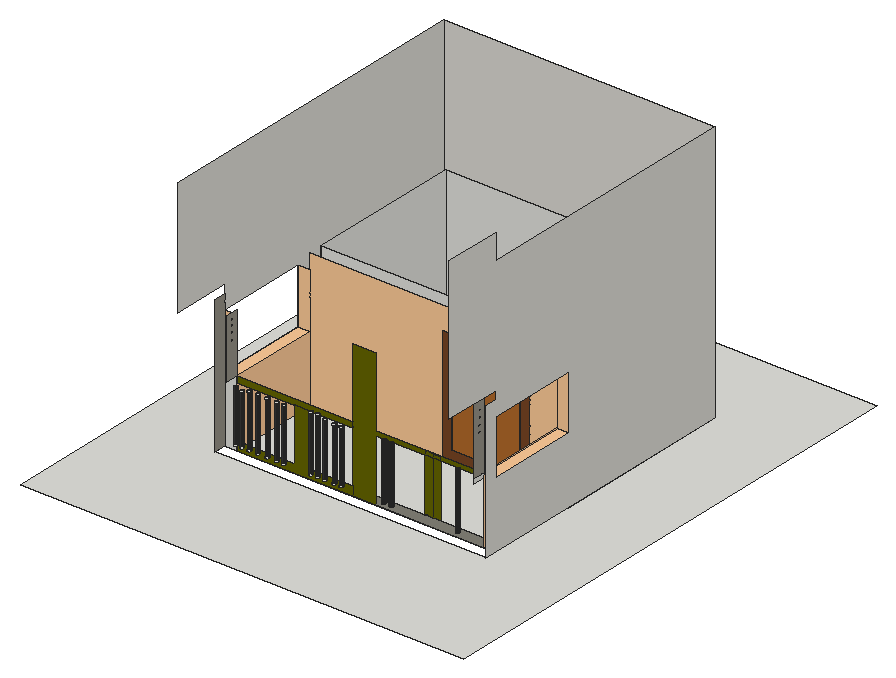
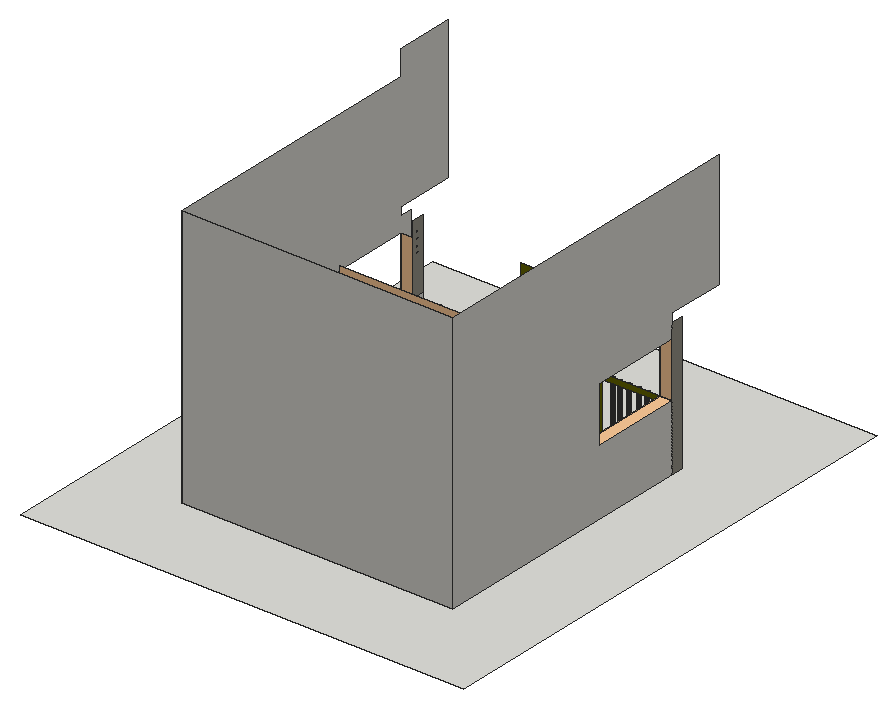
# SketchUp Ruby script. Lengths in inches.
U = 1.inch
M = Sketchup.active_model
def pt(a) = Geom::Point3d.new(a.map { |v| v * U })
def face(e, loops, mat)
  f = e.add_face(loops[0].map { |a| pt(a) })
  loops[1..].each { |l| e.add_face(l.map { |a| pt(a) }).erase! }
  f.material = f.back_material = mat if mat
  f
end
# faces: each face lists its corners as indices into pts; further lists are holes
def faces(e, pts, list, mat = nil) = list.each { |f| face(e, (f[0].is_a?(Array) ? f : [f]).map { |l| l.map { |i| pts[i] } }, mat) }
# xy, xz, yz: faces in a plane at the given z, y or x. An outline is a flat list of corners, or four numbers for a rectangle; further outlines are holes
def ring(l) = l.size == 4 ? [[l[0], l[1]], [l[2], l[1]], [l[2], l[3]], [l[0], l[3]]] : l.each_slice(2).to_a
def flat(e, list, mat, &to3) = list.each { |f| face(e, (f[0].is_a?(Array) ? f : [f]).map { |l| ring(l).map { |u, v| to3.(u, v) } }, mat) }
def xy(e, z, list, mat = nil) = flat(e, list, mat) { |x, y| [x, y, z] }
def xz(e, y, list, mat = nil) = flat(e, list, mat) { |x, z| [x, y, z] }
def yz(e, x, list, mat = nil) = flat(e, list, mat) { |y, z| [x, y, z] }
def lines(e, pts, list) = list.each { |a, b| e.add_line(pt(pts[a]), pt(pts[b])) }
# prism: a flat outline (further loops are holes) pulled along v
def prism(e, loops, v, mat = nil)
  f = face(e, loops, mat); d = Geom::Vector3d.new(v.map { |x| x * U })
  f.pushpull(f.normal.samedirection?(d) ? d.length : -d.length)
end
def box(e, o, s, mat = nil) = prism(e, [[o, [o[0] + s[0], o[1], o[2]], [o[0] + s[0], o[1] + s[1], o[2]], [o[0], o[1] + s[1], o[2]]]], [0, 0, s[2]], mat)
def at(x, y, z, deg = 0) = Geom::Transformation.translation(pt([x, y, z])) * Geom::Transformation.rotation(ORIGIN, Z_AXIS, deg.degrees)
def axes(o, x, y, z) = Geom::Transformation.new([*x, 0, *y, 0, *z, 0, *pt(o).to_a, 1])
def part(name) = M.definitions.add(name)
# library, detail: a bought-in or finely detailed component or shape, given as its bounding box
def library(name, o, s) = part(name).tap { |d| box(d.entities, o, s) }
def detail(e, o, s) = box(e.add_group.entities, o, s)
def put(e, d, t, mat = nil) = e.add_instance(d, t).tap { |i| i.material = mat if mat }
def group(e, t, mat = nil) = e.add_group.tap { |g| g.transformation = t; g.material = mat if mat }.entities
root = M.entities
M.materials.add("[Color C02]").color = [255, 204, 153]
M.materials.add("[Color E08]").color = [102, 102, 0]
M.materials.add("[Color M07]").color = [58, 58, 58]
M.materials.add("[Formica Graystone]").color = [149, 146, 135]
M.materials.add("[Terrazzo Tile Light]").color = [219, 217, 210]
M.materials.add("[Wood Bamboo]").color = [177, 105, 43]
M.materials.add("[Wood Veneer 01]").color = [120, 70, 37]
xy(root,0,[[[0,0,171.0625,199],[33.03,52.46,137.78,162.77]],[33.03,57.16,37.72,92.52],[37.72,57.16,133.09,92.52],[133.09,57.16,137.78,92.52],[[33.03,92.52,137.78,162.77],[37.72,98,133.09,158.08]],
  [37.72,98,133.09,158.08]])
xy(root,3.4375,[[39.18,54.27,39,54.29,38.83,54.36,38.69,54.47,38.58,54.61,38.51,54.78,38.49,54.96,38.51,55.13,38.58,55.3,38.69,55.44,38.83,55.55,39,55.62,39.18,55.64,39.35,55.62,39.52,55.55,39.66,55.44,39.77,55.3,39.84,55.13,39.86,54.96,39.84,54.78,39.77,54.61,39.66,54.47,39.52,54.36,39.35,54.29],[41.55,54.27,41.375,54.29,41.21,54.36,41.07,54.47,40.96,54.61,40.89,54.78,40.86,54.96,40.89,55.13,40.96,55.3,41.07,55.44,41.21,55.55,41.375,55.62,41.55,55.64,41.73,55.62,41.9,55.55,42.04,55.44,42.15,55.3,42.22,55.13,42.24,54.96,42.22,54.78,42.15,54.61,42.04,54.47,41.9,54.36,41.73,54.29],[44.43,54.27,44.25,54.29,44.08,54.36,43.94,54.47,43.83,54.61,43.76,54.78,43.74,54.96,43.76,55.13,43.83,55.3,43.94,55.44,44.08,55.55,44.25,55.62,44.43,55.64,44.6,55.62,44.77,55.55,44.91,55.44,45.02,55.3,45.09,55.13,45.11,54.96,45.09,54.78,45.02,54.61,44.91,54.47,44.77,54.36,44.6,54.29],[47.68,54.27,47.5,54.29,47.33,54.36,47.19,54.47,47.08,54.61,47.01,54.78,46.99,54.96,47.01,55.13,47.08,55.3,47.19,55.44,47.33,55.55,47.5,55.62,47.68,55.64,47.85,55.62,48.02,55.55,48.16,55.44,48.27,55.3,48.34,55.13,48.36,54.96,48.34,54.78,48.27,54.61,48.16,54.47,48.02,54.36,47.85,54.29],[51.36,54.27,51.1875,54.29,51.02,54.36,50.88,54.47,50.77,54.61,50.7,54.78,50.68,54.96,50.7,55.13,50.77,55.3,50.88,55.44,51.02,55.55,51.1875,55.62,51.36,55.64,51.54,55.62,51.71,55.55,51.85,55.44,51.96,55.3,52.03,55.13,52.05,54.96,52.03,54.78,51.96,54.61,51.85,54.47,51.71,54.36,51.54,54.29],
  [54.99,54.27,54.8125,54.29,54.65,54.36,54.5,54.47,54.39,54.61,54.32,54.78,54.3,54.96,54.32,55.13,54.39,55.3,54.5,55.44,54.65,55.55,54.8125,55.62,54.99,55.64,55.17,55.62,55.33,55.55,55.48,55.44,55.58,55.3,55.65,55.13,55.68,54.96,55.65,54.78,55.58,54.61,55.48,54.47,55.33,54.36,55.17,54.29],[57.74,54.27,57.5625,54.29,57.4,54.36,57.25,54.47,57.14,54.61,57.07,54.78,57.05,54.96,57.07,55.13,57.14,55.3,57.25,55.44,57.4,55.55,57.5625,55.62,57.74,55.64,57.92,55.62,58.08,55.55,58.23,55.44,58.33,55.3,58.4,55.13,58.43,54.96,58.4,54.78,58.33,54.61,58.23,54.47,58.08,54.36,57.92,54.29],[68.11,54.27,67.9375,54.29,67.77,54.36,67.63,54.47,67.52,54.61,67.45,54.78,67.43,54.96,67.45,55.13,67.52,55.3,67.63,55.44,67.77,55.55,67.9375,55.62,68.11,55.64,68.29,55.62,68.46,55.55,68.6,55.44,68.71,55.3,68.78,55.13,68.8,54.96,68.78,54.78,68.71,54.61,68.6,54.47,68.46,54.36,68.29,54.29],[70.74,54.27,70.5625,54.29,70.4,54.36,70.25,54.47,70.14,54.61,70.07,54.78,70.05,54.96,70.07,55.13,70.14,55.3,70.25,55.44,70.4,55.55,70.5625,55.62,70.74,55.64,70.92,55.62,71.08,55.55,71.23,55.44,71.33,55.3,71.4,55.13,71.43,54.96,71.4,54.78,71.33,54.61,71.23,54.47,71.08,54.36,70.92,54.29],[73.55,54.27,73.375,54.29,73.21,54.36,73.07,54.47,72.96,54.61,72.89,54.78,72.86,54.96,72.89,55.13,72.96,55.3,73.07,55.44,73.21,55.55,73.375,55.62,73.55,55.64,73.73,55.62,73.9,55.55,74.04,55.44,74.15,55.3,74.22,55.13,74.24,54.96,74.22,54.78,74.15,54.61,74.04,54.47,73.9,54.36,73.73,54.29],
  [77.18,54.27,77,54.29,76.83,54.36,76.69,54.47,76.58,54.61,76.51,54.78,76.49,54.96,76.51,55.13,76.58,55.3,76.69,55.44,76.83,55.55,77,55.62,77.18,55.64,77.35,55.62,77.52,55.55,77.66,55.44,77.77,55.3,77.84,55.13,77.86,54.96,77.84,54.78,77.77,54.61,77.66,54.47,77.52,54.36,77.35,54.29],[79.8,54.27,79.625,54.29,79.46,54.36,79.32,54.47,79.21,54.61,79.14,54.78,79.11,54.96,79.14,55.13,79.21,55.3,79.32,55.44,79.46,55.55,79.625,55.62,79.8,55.64,79.98,55.62,80.15,55.55,80.29,55.44,80.4,55.3,80.47,55.13,80.49,54.96,80.47,54.78,80.4,54.61,80.29,54.47,80.15,54.36,79.98,54.29]])
xy(root,3.82,[[92.4,92.52,118.56,98]])
xy(root,22.875,[[41.55,54.27,41.73,54.29,41.9,54.36,42.04,54.47,42.15,54.61,42.22,54.78,42.24,54.96,42.22,55.13,42.15,55.3,42.04,55.44,41.9,55.55,41.73,55.62,41.55,55.64,41.375,55.62,41.21,55.55,41.07,55.44,40.96,55.3,40.89,55.13,40.86,54.96,40.89,54.78,40.96,54.61,41.07,54.47,41.21,54.36,41.375,54.29]])
xy(root,23.8125,[[54.99,54.27,55.17,54.29,55.33,54.36,55.48,54.47,55.58,54.61,55.65,54.78,55.68,54.96,55.65,55.13,55.58,55.3,55.48,55.44,55.33,55.55,55.17,55.62,54.99,55.64,54.8125,55.62,54.65,55.55,54.5,55.44,54.39,55.3,54.32,55.13,54.3,54.96,54.32,54.78,54.39,54.61,54.5,54.47,54.65,54.36,54.8125,54.29]])
xy(root,23.875,[[44.43,54.27,44.6,54.29,44.77,54.36,44.91,54.47,45.02,54.61,45.09,54.78,45.11,54.96,45.09,55.13,45.02,55.3,44.91,55.44,44.77,55.55,44.6,55.62,44.43,55.64,44.25,55.62,44.08,55.55,43.94,55.44,43.83,55.3,43.76,55.13,43.74,54.96,43.76,54.78,43.83,54.61,43.94,54.47,44.08,54.36,44.25,54.29]])
xy(root,23.9375,[[47.68,54.27,47.85,54.29,48.02,54.36,48.16,54.47,48.27,54.61,48.34,54.78,48.36,54.96,48.34,55.13,48.27,55.3,48.16,55.44,48.02,55.55,47.85,55.62,47.68,55.64,47.5,55.62,47.33,55.55,47.19,55.44,47.08,55.3,47.01,55.13,46.99,54.96,47.01,54.78,47.08,54.61,47.19,54.47,47.33,54.36,47.5,54.29],[51.36,54.27,51.54,54.29,51.71,54.36,51.85,54.47,51.96,54.61,52.03,54.78,52.05,54.96,52.03,55.13,51.96,55.3,51.85,55.44,51.71,55.55,51.54,55.62,51.36,55.64,51.1875,55.62,51.02,55.55,50.88,55.44,50.77,55.3,50.7,55.13,50.68,54.96,50.7,54.78,50.77,54.61,50.88,54.47,51.02,54.36,51.1875,54.29],[57.74,54.27,57.92,54.29,58.08,54.36,58.23,54.47,58.33,54.61,58.4,54.78,58.43,54.96,58.4,55.13,58.33,55.3,58.23,55.44,58.08,55.55,57.92,55.62,57.74,55.64,57.5625,55.62,57.4,55.55,57.25,55.44,57.14,55.3,57.07,55.13,57.05,54.96,57.07,54.78,57.14,54.61,57.25,54.47,57.4,54.36,57.5625,54.29]])
xy(root,24,[[77.18,54.27,77.35,54.29,77.52,54.36,77.66,54.47,77.77,54.61,77.84,54.78,77.86,54.96,77.84,55.13,77.77,55.3,77.66,55.44,77.52,55.55,77.35,55.62,77.18,55.64,77,55.62,76.83,55.55,76.69,55.44,76.58,55.3,76.51,55.13,76.49,54.96,76.51,54.78,76.58,54.61,76.69,54.47,76.83,54.36,77,54.29]])
xy(root,24.0625,[[79.8,54.27,79.98,54.29,80.15,54.36,80.29,54.47,80.4,54.61,80.47,54.78,80.49,54.96,80.47,55.13,80.4,55.3,80.29,55.44,80.15,55.55,79.98,55.62,79.8,55.64,79.625,55.62,79.46,55.55,79.32,55.44,79.21,55.3,79.14,55.13,79.11,54.96,79.14,54.78,79.21,54.61,79.32,54.47,79.46,54.36,79.625,54.29]])
xy(root,24.375,[[73.55,54.27,73.73,54.29,73.9,54.36,74.04,54.47,74.15,54.61,74.22,54.78,74.24,54.96,74.22,55.13,74.15,55.3,74.04,55.44,73.9,55.55,73.73,55.62,73.55,55.64,73.375,55.62,73.21,55.55,73.07,55.44,72.96,55.3,72.89,55.13,72.86,54.96,72.89,54.78,72.96,54.61,73.07,54.47,73.21,54.36,73.375,54.29]])
xy(root,25.0625,[[68.11,54.27,68.29,54.29,68.46,54.36,68.6,54.47,68.71,54.61,68.78,54.78,68.8,54.96,68.78,55.13,68.71,55.3,68.6,55.44,68.46,55.55,68.29,55.62,68.11,55.64,67.9375,55.62,67.77,55.55,67.63,55.44,67.52,55.3,67.45,55.13,67.43,54.96,67.45,54.78,67.52,54.61,67.63,54.47,67.77,54.36,67.9375,54.29]])
xy(root,25.1875,[[70.74,54.27,70.92,54.29,71.08,54.36,71.23,54.47,71.33,54.61,71.4,54.78,71.43,54.96,71.4,55.13,71.33,55.3,71.23,55.44,71.08,55.55,70.92,55.62,70.74,55.64,70.5625,55.62,70.4,55.55,70.25,55.44,70.14,55.3,70.07,55.13,70.05,54.96,70.07,54.78,70.14,54.61,70.25,54.47,70.4,54.36,70.5625,54.29]])
xy(root,25.6875,[[33.03,57.16,37.72,92.52],[133.09,57.16,137.78,92.52]],"[Color C02]")
xz(root,57.16,[[33.03,0,37.72,25.6875],[110.32,3.25,113.44,3.4375]])
xz(root,57.16,[[33.03,25.6875,37.72,46.9375],[133.09,25.6875,137.78,46.9375]],"[Color C02]")
xz(root,57.16,[[37.72,0,37.72,3.4375,60.17,3.4375,60.17,23.55,65.76,23.55,65.76,3.4375,82.62,3.4375,82.62,0],[82.62,0,82.62,52.6875,91.56,52.6875,91.56,25.83,133.09,25.83,133.09,24.05,116.56,24.05,116.56,25.6875,110.32,25.6875,110.32,24.05,91.56,24.05,91.56,0],[110.32,3.4375,113.44,24.05],[113.44,3.4375,116.56,24.05],[37.72,23.55,82.62,25.6875],
  [110.32,24.05,113.44,25.6875],[113.44,24.05,116.56,25.6875]],"[Color E08]")
xz(root,57.16,[[91.56,0,91.56,3.4375,110.32,3.4375,110.32,3.25,113.44,3.25,113.44,3.4375,133.09,3.4375,133.09,0]],"[Formica Graystone]")
xz(root,92.52,[[37.72,0,88.58,0,88.58,44.125,122.39,44.125,122.39,0,133.09,0,133.09,52.6875,37.72,52.6875],[33.03,25.6875,37.72,46.9375],[133.09,25.6875,137.78,46.9375]],"[Color C02]")
xz(root,92.52,[[92.4,3.82,118.56,40.3]],"[Wood Bamboo]")
xz(root,92.52,[[[88.58,0,122.39,44.125],[92.4,3.82,118.56,40.3]]],"[Wood Veneer 01]")
xz(root,98,[[[37.72,0,133.09,52.6875],[92.4,3.82,118.56,40.3]]])
xz(root,158.08,[[37.72,0,133.09,52.6875]])
xz(root,162.77,[[33.03,0,137.78,100.8125]],"[Terrazzo Tile Light]")
yz(root,33.03,[[52.46,0,57.16,52.6875]],"[Formica Graystone]")
yz(root,33.03,[[57.16,0,57.16,25.6875,92.52,25.6875,92.52,46.9375,57.16,46.9375,57.16,55.875,34.66,55.875,34.66,100.8125,162.77,100.8125,162.77,0]],"[Terrazzo Tile Light]")
yz(root,37.72,[[98,0,158.08,52.6875]])
yz(root,37.72,[[57.16,0,92.52,25.6875]],"[Color C02]")
yz(root,37.72,[[[52.46,25.6875,57.16,48.59],[54.84,45.92,54.69,45.94,54.56,46,54.44,46.09,54.35,46.2,54.3,46.34,54.28,46.48,54.3,46.63,54.35,46.77,54.44,46.88,54.56,46.97,54.69,47.03,54.84,47.05,54.99,47.03,55.12,46.97,55.24,46.88,55.33,46.77,55.38,46.63,55.4,46.48,55.38,46.34,55.33,46.2,55.24,46.09,55.12,46,54.99,45.94],[54.84,38.61,54.69,38.63,54.56,38.68,54.44,38.77,54.35,38.89,54.3,39.03,54.28,39.17,54.3,39.32,54.35,39.45,54.44,39.57,54.56,39.66,54.69,39.72,54.84,39.73,54.99,39.72,55.12,39.66,55.24,39.57,55.33,39.45,55.38,39.32,55.4,39.17,55.38,39.03,55.33,38.89,55.24,38.77,55.12,38.68,54.99,38.63],[54.84,41.36,54.69,41.38,54.56,41.43,54.44,41.52,54.35,41.64,54.3,41.78,54.28,41.92,54.3,42.07,54.35,42.2,54.44,42.32,54.56,42.41,54.69,42.47,54.84,42.48,54.99,42.47,55.12,42.41,55.24,42.32,55.33,42.2,55.38,42.07,55.4,41.92,55.38,41.78,55.33,41.64,55.24,41.52,55.12,41.43,54.99,41.38],[54.84,43.67,54.69,43.69,54.56,43.75,54.44,43.84,54.35,43.95,54.3,44.09,54.28,44.23,54.3,44.38,54.35,44.52,54.44,44.63,54.56,44.72,54.69,44.78,54.84,44.8,54.99,44.78,55.12,44.72,55.24,44.63,55.33,44.52,55.38,44.38,55.4,44.23,55.38,44.09,55.33,43.95,55.24,43.84,55.12,43.75,54.99,43.69]]],"[Formica Graystone]")
yz(root,92.4,[[92.52,3.82,98,40.3]])
yz(root,118.56,[[92.52,3.82,98,40.3]])
yz(root,133.09,[[98,0,158.08,52.6875],[52.46,24.05,57.16,25.83]])
yz(root,133.09,[[57.16,0,92.52,25.6875]],"[Color C02]")
yz(root,133.09,[[[52.46,25.83,57.16,52.6875],[55.04,40.18,55.1875,40.2,55.32,40.26,55.4375,40.35,55.53,40.46,55.58,40.6,55.6,40.75,55.58,40.89,55.53,41.03,55.4375,41.14,55.32,41.23,55.1875,41.29,55.04,41.31,54.9,41.29,54.76,41.23,54.64,41.14,54.55,41.03,54.5,40.89,54.48,40.75,54.5,40.6,54.55,40.46,54.64,40.35,54.76,40.26,54.9,40.2],[55.04,42.56,55.1875,42.58,55.32,42.63,55.4375,42.72,55.53,42.84,55.58,42.98,55.6,43.12,55.58,43.27,55.53,43.4,55.4375,43.52,55.32,43.61,55.1875,43.66,55.04,43.68,54.9,43.66,54.76,43.61,54.64,43.52,54.55,43.4,54.5,43.27,54.48,43.12,54.5,42.98,54.55,42.84,54.64,42.72,54.76,42.63,54.9,42.58],[55.04,45.18,55.1875,45.2,55.32,45.26,55.4375,45.35,55.53,45.46,55.58,45.6,55.6,45.75,55.58,45.89,55.53,46.03,55.4375,46.14,55.32,46.23,55.1875,46.29,55.04,46.31,54.9,46.29,54.76,46.23,54.64,46.14,54.55,46.03,54.5,45.89,54.48,45.75,54.5,45.6,54.55,45.46,54.64,45.35,54.76,45.26,54.9,45.2],[55.04,47.68,55.1875,47.7,55.32,47.76,55.4375,47.85,55.53,47.96,55.58,48.1,55.6,48.25,55.58,48.39,55.53,48.53,55.4375,48.64,55.32,48.73,55.1875,48.79,55.04,48.81,54.9,48.79,54.76,48.73,54.64,48.64,54.55,48.53,54.5,48.39,54.48,48.25,54.5,48.1,54.55,47.96,54.64,47.85,54.76,47.76,54.9,47.7]]],"[Formica Graystone]")
yz(root,137.78,[[52.46,0,162.77,0,162.77,100.8125,57.16,100.8125,57.16,110.5625,34.66,110.5625,34.66,55.875,57.16,55.875,57.16,46.9375,92.52,46.9375,92.52,25.6875,57.16,25.6875,57.16,52.6875,52.46,52.6875]],"[Terrazzo Tile Light]")
p = [[96.08,54.36,3.4375],[96.25,54.29,3.4375],[96.25,54.29,25.1875],[96.08,54.36,25.1875],[96.43,54.27,3.4375],[96.43,54.27,25.1875],
  [96.6,54.29,3.4375],[96.6,54.29,25.1875],[96.77,54.36,3.4375],[96.77,54.36,25.1875],[98.9,54.36,3.4375],[99.0625,54.29,3.4375],
  [99.0625,54.29,25.1875],[98.9,54.36,25.1875],[99.24,54.27,3.4375],[99.24,54.27,25.1875],[99.42,54.29,3.4375],[99.42,54.29,25.1875],
  [99.58,54.36,3.4375],[99.58,54.36,25.1875],[124.46,54.36,3.4375],[124.625,54.29,3.4375],[124.625,54.29,25.1875],[124.46,54.36,25.1875],
  [124.8,54.27,3.4375],[124.8,54.27,25.1875],[124.98,54.29,3.4375],[124.98,54.29,25.1875],[125.15,54.36,3.4375],[125.15,54.36,25.1875],
  [95.94,54.47,3.4375],[95.94,54.47,25.1875],[96.91,54.47,3.4375],[96.91,54.47,25.1875],[98.75,54.47,3.4375],[98.75,54.47,25.1875],
  [99.73,54.47,3.4375],[99.73,54.47,25.1875],[124.32,54.47,3.4375],[124.32,54.47,25.1875],[125.29,54.47,3.4375],[125.29,54.47,25.1875],
  [95.83,54.61,3.4375],[95.83,54.61,25.1875],[97.02,54.61,3.4375],[97.02,54.61,25.1875],[98.64,54.61,3.4375],[98.64,54.61,25.1875],
  [99.83,54.61,3.4375],[99.83,54.61,25.1875],[124.21,54.61,3.4375],[124.21,54.61,25.1875],[125.4,54.61,3.4375],[125.4,54.61,25.1875],
  [95.76,54.78,3.4375],[95.76,54.78,25.1875],[97.09,54.78,3.4375],[97.09,54.78,25.1875],[98.57,54.78,3.4375],[98.57,54.78,25.1875],
  [99.9,54.78,3.4375],[99.9,54.78,25.1875],[124.14,54.78,3.4375],[124.14,54.78,25.1875],[125.47,54.78,3.4375],[125.47,54.78,25.1875],
  [95.74,54.96,3.4375],[95.74,54.96,25.1875],[97.11,54.96,3.4375],[97.11,54.96,25.1875],[98.55,54.96,3.4375],[98.55,54.96,25.1875],
  [99.93,54.96,3.4375],[99.93,54.96,25.1875],[124.11,54.96,3.4375],[124.11,54.96,25.1875],[125.49,54.96,3.4375],[125.49,54.96,25.1875],
  [38.51,55.13,3.4375],[38.49,54.96,3.4375],[38.49,54.96,23.55],[38.51,55.13,23.55],[39.86,54.96,3.4375],[39.84,55.13,3.4375],
  [39.84,55.13,23.55],[39.86,54.96,23.55],[40.89,55.13,3.4375],[40.86,54.96,3.4375],[40.86,54.96,22.875],[40.89,55.13,22.875],
  [42.24,54.96,3.4375],[42.22,55.13,3.4375],[42.22,55.13,22.875],[42.24,54.96,22.875],[43.76,55.13,3.4375],[43.74,54.96,3.4375],
  [43.74,54.96,23.875],[43.76,55.13,23.875],[45.11,54.96,3.4375],[45.09,55.13,3.4375],[45.09,55.13,23.875],[45.11,54.96,23.875],
  [47.01,55.13,3.4375],[46.99,54.96,3.4375],[46.99,54.96,23.9375],[47.01,55.13,23.9375],[48.36,54.96,3.4375],[48.34,55.13,3.4375],
  [48.34,55.13,23.9375],[48.36,54.96,23.9375],[50.7,55.13,3.4375],[50.68,54.96,3.4375],[50.68,54.96,23.9375],[50.7,55.13,23.9375],
  [52.05,54.96,3.4375],[52.03,55.13,3.4375],[52.03,55.13,23.9375],[52.05,54.96,23.9375],[54.32,55.13,3.4375],[54.3,54.96,3.4375],
  [54.3,54.96,23.8125],[54.32,55.13,23.8125],[55.68,54.96,3.4375],[55.65,55.13,3.4375],[55.65,55.13,23.8125],[55.68,54.96,23.8125],
  [57.07,55.13,3.4375],[57.05,54.96,3.4375],[57.05,54.96,23.9375],[57.07,55.13,23.9375],[58.43,54.96,3.4375],[58.4,55.13,3.4375],
  [58.4,55.13,23.9375],[58.43,54.96,23.9375],[67.45,55.13,3.4375],[67.43,54.96,3.4375],[67.43,54.96,25.0625],[67.45,55.13,25.0625],
  [68.8,54.96,3.4375],[68.78,55.13,3.4375],[68.78,55.13,25.0625],[68.8,54.96,25.0625],[70.07,55.13,3.4375],[70.05,54.96,3.4375],
  [70.05,54.96,25.1875],[70.07,55.13,25.1875],[71.43,54.96,3.4375],[71.4,55.13,3.4375],[71.4,55.13,25.1875],[71.43,54.96,25.1875],
  [72.89,55.13,3.4375],[72.86,54.96,3.4375],[72.86,54.96,24.375],[72.89,55.13,24.375],[74.24,54.96,3.4375],[74.22,55.13,3.4375],
  [74.22,55.13,24.375],[74.24,54.96,24.375],[76.51,55.13,3.4375],[76.49,54.96,3.4375],[76.49,54.96,24],[76.51,55.13,24],
  [77.86,54.96,3.4375],[77.84,55.13,3.4375],[77.84,55.13,24],[77.86,54.96,24],[79.14,55.13,3.4375],[79.11,54.96,3.4375],
  [79.11,54.96,24.0625],[79.14,55.13,24.0625],[80.49,54.96,3.4375],[80.47,55.13,3.4375],[80.47,55.13,24.0625],[80.49,54.96,24.0625],
  [95.76,55.13,3.4375],[95.76,55.13,25.1875],[97.09,55.13,3.4375],[97.09,55.13,25.1875],[98.57,55.13,3.4375],[98.57,55.13,25.1875],
  [99.9,55.13,3.4375],[99.9,55.13,25.1875],[124.14,55.13,3.4375],[124.14,55.13,25.1875],[125.47,55.13,3.4375],[125.47,55.13,25.1875],
  [38.58,55.3,3.4375],[38.58,55.3,23.55],[39.77,55.3,3.4375],[39.77,55.3,23.55],[40.96,55.3,3.4375],[40.96,55.3,22.875],
  [42.15,55.3,3.4375],[42.15,55.3,22.875],[43.83,55.3,3.4375],[43.83,55.3,23.875],[45.02,55.3,3.4375],[45.02,55.3,23.875],
  [47.08,55.3,3.4375],[47.08,55.3,23.9375],[48.27,55.3,3.4375],[48.27,55.3,23.9375],[50.77,55.3,3.4375],[50.77,55.3,23.9375],
  [51.96,55.3,3.4375],[51.96,55.3,23.9375],[54.39,55.3,3.4375],[54.39,55.3,23.8125],[55.58,55.3,3.4375],[55.58,55.3,23.8125],
  [57.14,55.3,3.4375],[57.14,55.3,23.9375],[58.33,55.3,3.4375],[58.33,55.3,23.9375],[67.52,55.3,3.4375],[67.52,55.3,25.0625],
  [68.71,55.3,3.4375],[68.71,55.3,25.0625],[70.14,55.3,3.4375],[70.14,55.3,25.1875],[71.33,55.3,3.4375],[71.33,55.3,25.1875],
  [72.96,55.3,3.4375],[72.96,55.3,24.375],[74.15,55.3,3.4375],[74.15,55.3,24.375],[76.58,55.3,3.4375],[76.58,55.3,24],
  [77.77,55.3,3.4375],[77.77,55.3,24],[79.21,55.3,3.4375],[79.21,55.3,24.0625],[80.4,55.3,3.4375],[80.4,55.3,24.0625],
  [95.83,55.3,3.4375],[95.83,55.3,25.1875],[97.02,55.3,3.4375],[97.02,55.3,25.1875],[98.64,55.3,3.4375],[98.64,55.3,25.1875],
  [99.83,55.3,3.4375],[99.83,55.3,25.1875],[124.21,55.3,3.4375],[124.21,55.3,25.1875],[125.4,55.3,3.4375],[125.4,55.3,25.1875],
  [38.69,55.44,3.4375],[38.69,55.44,23.55],[39.66,55.44,3.4375],[39.66,55.44,23.55],[41.07,55.44,3.4375],[41.07,55.44,22.875],
  [42.04,55.44,3.4375],[42.04,55.44,22.875],[43.94,55.44,3.4375],[43.94,55.44,23.875],[44.91,55.44,3.4375],[44.91,55.44,23.875],
  [47.19,55.44,3.4375],[47.19,55.44,23.9375],[48.16,55.44,3.4375],[48.16,55.44,23.9375],[50.88,55.44,3.4375],[50.88,55.44,23.9375],
  [51.85,55.44,3.4375],[51.85,55.44,23.9375],[54.5,55.44,3.4375],[54.5,55.44,23.8125],[55.48,55.44,3.4375],[55.48,55.44,23.8125],
  [57.25,55.44,3.4375],[57.25,55.44,23.9375],[58.23,55.44,3.4375],[58.23,55.44,23.9375],[67.63,55.44,3.4375],[67.63,55.44,25.0625],
  [68.6,55.44,3.4375],[68.6,55.44,25.0625],[70.25,55.44,3.4375],[70.25,55.44,25.1875],[71.23,55.44,3.4375],[71.23,55.44,25.1875],
  [73.07,55.44,3.4375],[73.07,55.44,24.375],[74.04,55.44,3.4375],[74.04,55.44,24.375],[76.69,55.44,3.4375],[76.69,55.44,24],
  [77.66,55.44,3.4375],[77.66,55.44,24],[79.32,55.44,3.4375],[79.32,55.44,24.0625],[80.29,55.44,3.4375],[80.29,55.44,24.0625],
  [95.94,55.44,3.4375],[95.94,55.44,25.1875],[96.91,55.44,3.4375],[96.91,55.44,25.1875],[98.75,55.44,3.4375],[98.75,55.44,25.1875],
  [99.73,55.44,3.4375],[99.73,55.44,25.1875],[124.32,55.44,3.4375],[124.32,55.44,25.1875],[125.29,55.44,3.4375],[125.29,55.44,25.1875],
  [38.83,55.55,3.4375],[38.83,55.55,23.55],[39.52,55.55,3.4375],[39.52,55.55,23.55],[41.21,55.55,3.4375],[41.21,55.55,22.875],
  [41.9,55.55,3.4375],[41.9,55.55,22.875],[44.08,55.55,3.4375],[44.08,55.55,23.875],[44.77,55.55,3.4375],[44.77,55.55,23.875],
  [47.33,55.55,3.4375],[47.33,55.55,23.9375],[48.02,55.55,3.4375],[48.02,55.55,23.9375],[51.02,55.55,3.4375],[51.02,55.55,23.9375],
  [51.71,55.55,3.4375],[51.71,55.55,23.9375],[54.65,55.55,3.4375],[54.65,55.55,23.8125],[55.33,55.55,3.4375],[55.33,55.55,23.8125],
  [57.4,55.55,3.4375],[57.4,55.55,23.9375],[58.08,55.55,3.4375],[58.08,55.55,23.9375],[67.77,55.55,3.4375],[67.77,55.55,25.0625],
  [68.46,55.55,3.4375],[68.46,55.55,25.0625],[70.4,55.55,3.4375],[70.4,55.55,25.1875],[71.08,55.55,3.4375],[71.08,55.55,25.1875],
  [73.21,55.55,3.4375],[73.21,55.55,24.375],[73.9,55.55,3.4375],[73.9,55.55,24.375],[76.83,55.55,3.4375],[76.83,55.55,24],
  [77.52,55.55,3.4375],[77.52,55.55,24],[79.46,55.55,3.4375],[79.46,55.55,24.0625],[80.15,55.55,3.4375],[80.15,55.55,24.0625],
  [96.08,55.55,3.4375],[96.08,55.55,25.1875],[96.77,55.55,3.4375],[96.77,55.55,25.1875],[98.9,55.55,3.4375],[98.9,55.55,25.1875],
  [99.58,55.55,3.4375],[99.58,55.55,25.1875],[124.46,55.55,3.4375],[124.46,55.55,25.1875],[125.15,55.55,3.4375],[125.15,55.55,25.1875],
  [39,55.62,3.4375],[39,55.62,23.55],[39.18,55.64,3.4375],[39.18,55.64,23.55],[39.35,55.62,3.4375],[39.35,55.62,23.55],
  [41.375,55.62,3.4375],[41.375,55.62,22.875],[41.55,55.64,3.4375],[41.55,55.64,22.875],[41.73,55.62,3.4375],[41.73,55.62,22.875],
  [44.25,55.62,3.4375],[44.25,55.62,23.875],[44.43,55.64,3.4375],[44.43,55.64,23.875],[44.6,55.62,3.4375],[44.6,55.62,23.875],
  [47.5,55.62,3.4375],[47.5,55.62,23.9375],[47.68,55.64,3.4375],[47.68,55.64,23.9375],[47.85,55.62,3.4375],[47.85,55.62,23.9375],
  [51.1875,55.62,3.4375],[51.1875,55.62,23.9375],[51.36,55.64,3.4375],[51.36,55.64,23.9375],[51.54,55.62,3.4375],[51.54,55.62,23.9375],
  [54.8125,55.62,3.4375],[54.8125,55.62,23.8125],[54.99,55.64,3.4375],[54.99,55.64,23.8125],[55.17,55.62,3.4375],[55.17,55.62,23.8125],
  [57.5625,55.62,3.4375],[57.5625,55.62,23.9375],[57.74,55.64,3.4375],[57.74,55.64,23.9375],[57.92,55.62,3.4375],[57.92,55.62,23.9375],
  [67.9375,55.62,3.4375],[67.9375,55.62,25.0625],[68.11,55.64,3.4375],[68.11,55.64,25.0625],[68.29,55.62,3.4375],[68.29,55.62,25.0625],
  [70.5625,55.62,3.4375],[70.5625,55.62,25.1875],[70.74,55.64,3.4375],[70.74,55.64,25.1875],[70.92,55.62,3.4375],[70.92,55.62,25.1875],
  [73.375,55.62,3.4375],[73.375,55.62,24.375],[73.55,55.64,3.4375],[73.55,55.64,24.375],[73.73,55.62,3.4375],[73.73,55.62,24.375],
  [77,55.62,3.4375],[77,55.62,24],[77.18,55.64,3.4375],[77.18,55.64,24],[77.35,55.62,3.4375],[77.35,55.62,24],
  [79.625,55.62,3.4375],[79.625,55.62,24.0625],[79.8,55.64,3.4375],[79.8,55.64,24.0625],[79.98,55.62,3.4375],[79.98,55.62,24.0625],
  [96.25,55.62,3.4375],[96.25,55.62,25.1875],[96.43,55.64,3.4375],[96.43,55.64,25.1875],[96.6,55.62,3.4375],[96.6,55.62,25.1875],
  [99.0625,55.62,3.4375],[99.0625,55.62,25.1875],[99.24,55.64,3.4375],[99.24,55.64,25.1875],[99.42,55.62,3.4375],[99.42,55.62,25.1875],
  [124.625,55.62,3.4375],[124.625,55.62,25.1875],[124.8,55.64,3.4375],[124.8,55.64,25.1875],[124.98,55.62,3.4375],[124.98,55.62,25.1875]]
faces(root,p,[[0,1,2,3],[1,4,5,2],[4,6,7,5],[6,8,9,7],[10,11,12,13],[11,14,15,12],[14,16,17,15],[16,18,19,17],
  [20,21,22,23],[21,24,25,22],[24,26,27,25],[26,28,29,27],[30,0,3,31],[8,32,33,9],[34,10,13,35],[18,36,37,19],
  [38,20,23,39],[28,40,41,29],[42,30,31,43],[32,44,45,33],[46,34,35,47],[36,48,49,37],[50,38,39,51],[40,52,53,41],
  [54,42,43,55],[44,56,57,45],[58,46,47,59],[48,60,61,49],[62,50,51,63],[52,64,65,53],[66,54,55,67],[56,68,69,57],
  [70,58,59,71],[60,72,73,61],[74,62,63,75],[64,76,77,65],[78,79,80,81],[82,83,84,85],[86,87,88,89],[90,91,92,93],
  [94,95,96,97],[98,99,100,101],[102,103,104,105],[106,107,108,109],[110,111,112,113],[114,115,116,117],[118,119,120,121],[122,123,124,125],
  [126,127,128,129],[130,131,132,133],[134,135,136,137],[138,139,140,141],[142,143,144,145],[146,147,148,149],[150,151,152,153],[154,155,156,157],
  [158,159,160,161],[162,163,164,165],[166,167,168,169],[170,171,172,173],[174,66,67,175],[68,176,177,69],[178,70,71,179],[72,180,181,73],
  [182,74,75,183],[76,184,185,77],[186,78,81,187],[83,188,189,84],[190,86,89,191],[91,192,193,92],[194,94,97,195],[99,196,197,100],
  [198,102,105,199],[107,200,201,108],[202,110,113,203],[115,204,205,116],[206,118,121,207],[123,208,209,124],[210,126,129,211],[131,212,213,132],
  [214,134,137,215],[139,216,217,140],[218,142,145,219],[147,220,221,148],[222,150,153,223],[155,224,225,156],[226,158,161,227],[163,228,229,164],
  [230,166,169,231],[171,232,233,172],[234,174,175,235],[176,236,237,177],[238,178,179,239],[180,240,241,181],[242,182,183,243],[184,244,245,185],
  [246,186,187,247],[188,248,249,189],[250,190,191,251],[192,252,253,193],[254,194,195,255],[196,256,257,197],[258,198,199,259],[200,260,261,201],
  [262,202,203,263],[204,264,265,205],[266,206,207,267],[208,268,269,209],[270,210,211,271],[212,272,273,213],[274,214,215,275],[216,276,277,217],
  [278,218,219,279],[220,280,281,221],[282,222,223,283],[224,284,285,225],[286,226,227,287],[228,288,289,229],[290,230,231,291],[232,292,293,233],
  [294,234,235,295],[236,296,297,237],[298,238,239,299],[240,300,301,241],[302,242,243,303],[244,304,305,245],[306,246,247,307],[248,308,309,249],
  [310,250,251,311],[252,312,313,253],[314,254,255,315],[256,316,317,257],[318,258,259,319],[260,320,321,261],[322,262,263,323],[264,324,325,265],
  [326,266,267,327],[268,328,329,269],[330,270,271,331],[272,332,333,273],[334,274,275,335],[276,336,337,277],[338,278,279,339],[280,340,341,281],
  [342,282,283,343],[284,344,345,285],[346,286,287,347],[288,348,349,289],[350,290,291,351],[292,352,353,293],[354,294,295,355],[296,356,357,297],
  [358,298,299,359],[300,360,361,301],[362,302,303,363],[304,364,365,305],[366,306,307,367],[368,366,367,369],[370,368,369,371],[308,370,371,309],
  [372,310,311,373],[374,372,373,375],[376,374,375,377],[312,376,377,313],[378,314,315,379],[380,378,379,381],[382,380,381,383],[316,382,383,317],
  [384,318,319,385],[386,384,385,387],[388,386,387,389],[320,388,389,321],[390,322,323,391],[392,390,391,393],[394,392,393,395],[324,394,395,325],
  [396,326,327,397],[398,396,397,399],[400,398,399,401],[328,400,401,329],[402,330,331,403],[404,402,403,405],[406,404,405,407],[332,406,407,333],
  [408,334,335,409],[410,408,409,411],[412,410,411,413],[336,412,413,337],[414,338,339,415],[416,414,415,417],[418,416,417,419],[340,418,419,341],
  [420,342,343,421],[422,420,421,423],[424,422,423,425],[344,424,425,345],[426,346,347,427],[428,426,427,429],[430,428,429,431],[348,430,431,349],
  [432,350,351,433],[434,432,433,435],[436,434,435,437],[352,436,437,353],[438,354,355,439],[440,438,439,441],[442,440,441,443],[356,442,443,357],
  [444,358,359,445],[446,444,445,447],[448,446,447,449],[360,448,449,361],[450,362,363,451],[452,450,451,453],[454,452,453,455],[364,454,455,365]],"[Color M07]")
